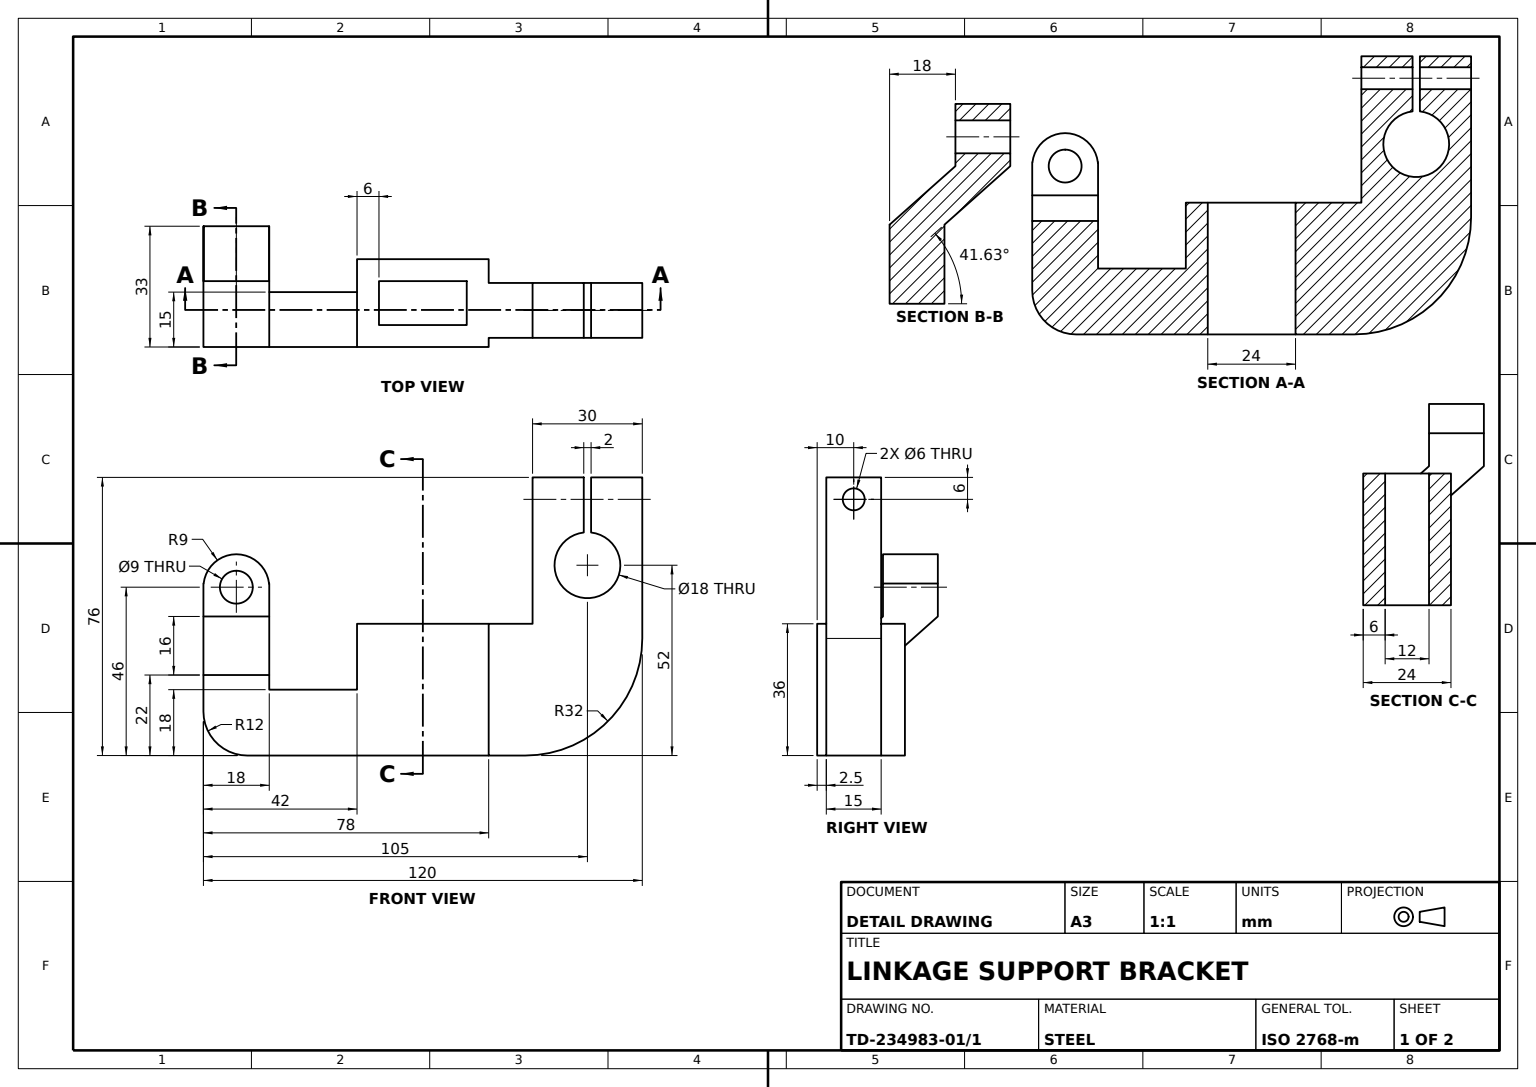
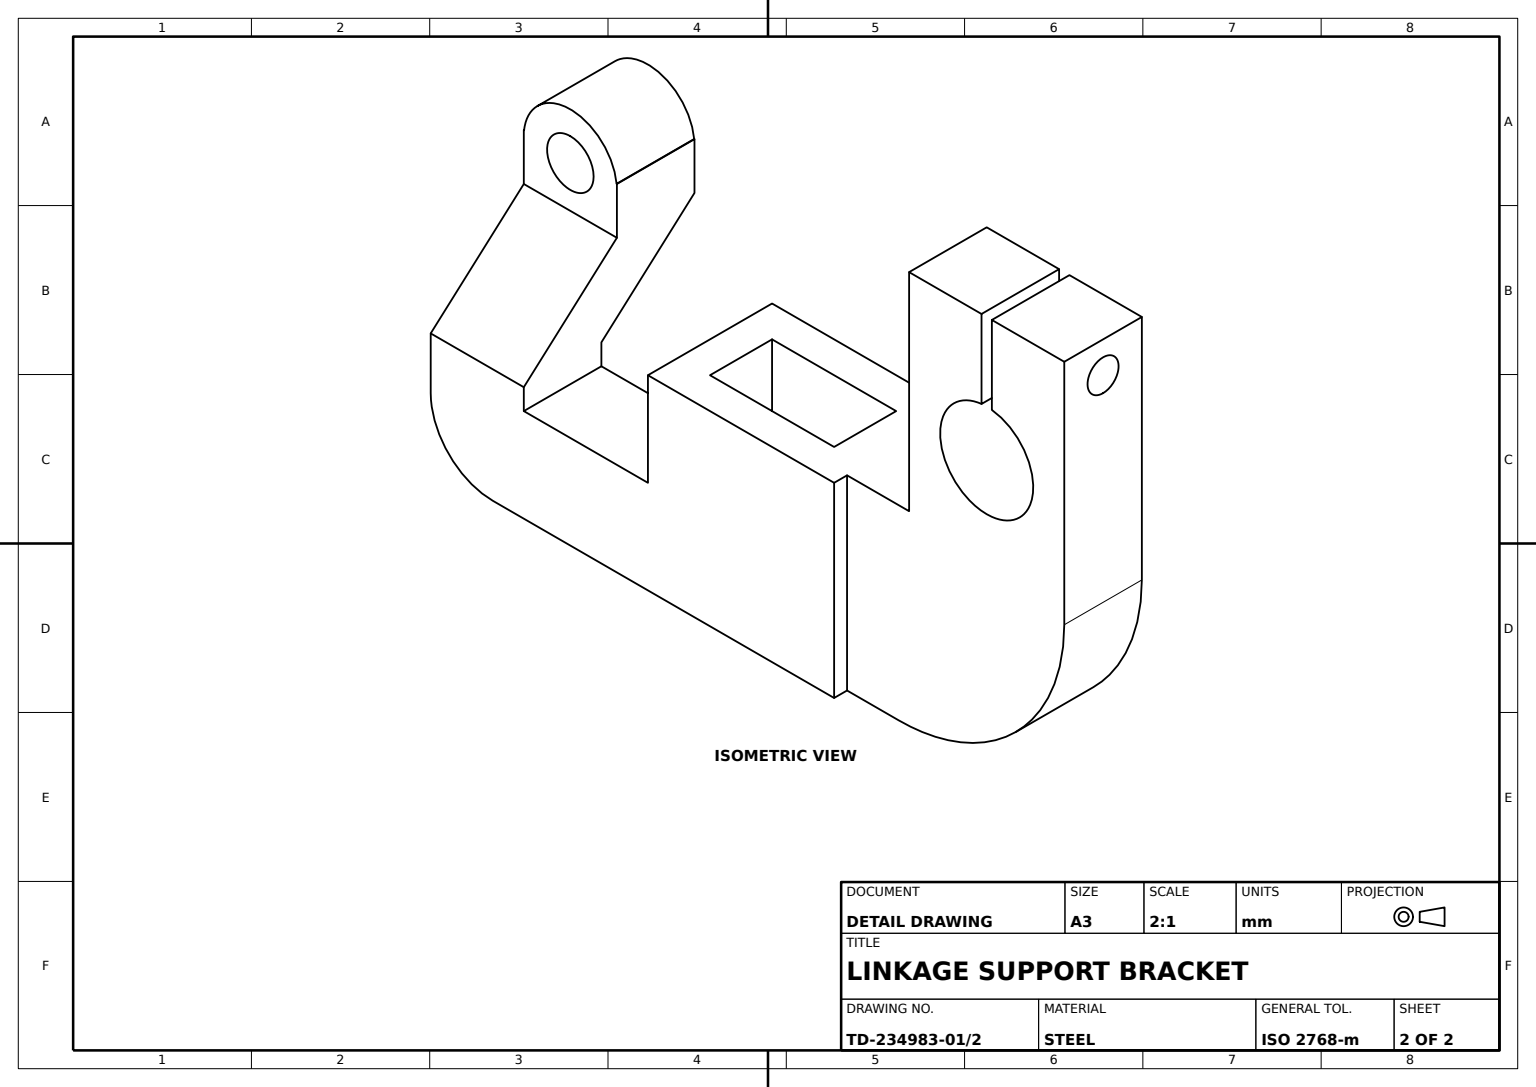
ISO-10303-21;
HEADER;
FILE_DESCRIPTION((''),'2;1');
FILE_NAME('','',(''),(''),'','','');
FILE_SCHEMA(('AUTOMOTIVE_DESIGN'));
ENDSEC;
DATA;
#1=APPLICATION_CONTEXT('');
#2=PRODUCT_CONTEXT('',#1,'mechanical');
#3=PRODUCT('','','',(#2));
#4=PRODUCT_DEFINITION_FORMATION('','',#3);
#5=PRODUCT_DEFINITION_CONTEXT('',#1,'design');
#6=PRODUCT_DEFINITION('','',#4,#5);
#7=PRODUCT_DEFINITION_SHAPE('','',#6);
#8=(LENGTH_UNIT()NAMED_UNIT(*)SI_UNIT(.MILLI.,.METRE.));
#9=(NAMED_UNIT(*)PLANE_ANGLE_UNIT()SI_UNIT($,.RADIAN.));
#10=(NAMED_UNIT(*)SI_UNIT($,.STERADIAN.)SOLID_ANGLE_UNIT());
#11=UNCERTAINTY_MEASURE_WITH_UNIT(LENGTH_MEASURE(0.005),#8,'distance_accuracy_value','');
#12=(GEOMETRIC_REPRESENTATION_CONTEXT(3)GLOBAL_UNCERTAINTY_ASSIGNED_CONTEXT((#11))GLOBAL_UNIT_ASSIGNED_CONTEXT((#8,#9,#10))REPRESENTATION_CONTEXT('',''));
#13=CARTESIAN_POINT('',(-16.5,18.,0.));
#14=VERTEX_POINT('',#13);
#15=CARTESIAN_POINT('',(-16.5,-18.,0.));
#16=VERTEX_POINT('',#15);
#17=DIRECTION('',(0.,-1.,0.));
#18=VECTOR('',#17,1000.);
#19=LINE('',#13,#18);
#20=EDGE_CURVE('',#14,#16,#19,.T.);
#21=ORIENTED_EDGE('',*,*,#20,.T.);
#22=CARTESIAN_POINT('',(-16.5,-18.,36.));
#23=VERTEX_POINT('',#22);
#24=DIRECTION('',(0.,0.,1.));
#25=VECTOR('',#24,1000.);
#26=LINE('',#15,#25);
#27=EDGE_CURVE('',#16,#23,#26,.T.);
#28=ORIENTED_EDGE('',*,*,#27,.T.);
#29=CARTESIAN_POINT('',(-16.5,18.,36.));
#30=VERTEX_POINT('',#29);
#31=DIRECTION('',(0.,1.,0.));
#32=VECTOR('',#31,1000.);
#33=LINE('',#22,#32);
#34=EDGE_CURVE('',#23,#30,#33,.T.);
#35=ORIENTED_EDGE('',*,*,#34,.T.);
#36=DIRECTION('',(0.,0.,-1.));
#37=VECTOR('',#36,1000.);
#38=LINE('',#29,#37);
#39=EDGE_CURVE('',#30,#14,#38,.T.);
#40=ORIENTED_EDGE('',*,*,#39,.T.);
#41=EDGE_LOOP('',(#21,#28,#35,#40));
#42=FACE_BOUND('',#41,.T.);
#43=CARTESIAN_POINT('',(-16.5,0.,0.));
#44=DIRECTION('',(-1.,0.,0.));
#45=AXIS2_PLACEMENT_3D('',#43,#44,#24);
#46=PLANE('',#45);
#47=ADVANCED_FACE('',(#42),#46,.T.);
#48=CARTESIAN_POINT('',(-25.5,-42.055728,47.));
#49=VERTEX_POINT('',#48);
#50=CARTESIAN_POINT('',(-25.5,-42.,47.));
#51=VERTEX_POINT('',#50);
#52=CARTESIAN_POINT('',(-25.5,-60.,47.));
#53=LINE('',#52,#32);
#54=EDGE_CURVE('',#49,#51,#53,.T.);
#55=ORIENTED_EDGE('',*,*,#54,.T.);
#56=CARTESIAN_POINT('',(-25.5,-42.,38.));
#57=VERTEX_POINT('',#56);
#58=LINE('',#56,#25);
#59=EDGE_CURVE('',#57,#51,#58,.T.);
#60=ORIENTED_EDGE('',*,*,#59,.F.);
#61=CARTESIAN_POINT('',(-25.5,-60.,38.));
#62=VERTEX_POINT('',#61);
#63=LINE('',#61,#32);
#64=EDGE_CURVE('',#62,#57,#63,.T.);
#65=ORIENTED_EDGE('',*,*,#64,.F.);
#66=VERTEX_POINT('',#52);
#67=LINE('',#61,#25);
#68=EDGE_CURVE('',#62,#66,#67,.T.);
#69=ORIENTED_EDGE('',*,*,#68,.T.);
#70=CARTESIAN_POINT('',(-25.5,-59.944272,47.));
#71=VERTEX_POINT('',#70);
#72=EDGE_CURVE('',#66,#71,#53,.T.);
#73=ORIENTED_EDGE('',*,*,#72,.T.);
#74=CARTESIAN_POINT('',(-25.5,-51.,46.));
#75=DIRECTION('',(1.,0.,0.));
#76=AXIS2_PLACEMENT_3D('',#74,#75,#31);
#77=CIRCLE('',#76,9.);
#78=EDGE_CURVE('',#49,#71,#77,.T.);
#79=ORIENTED_EDGE('',*,*,#78,.F.);
#80=EDGE_LOOP('',(#55,#60,#65,#69,#73,#79));
#81=FACE_BOUND('',#80,.T.);
#82=CARTESIAN_POINT('',(-25.5,-51.,50.5));
#83=VERTEX_POINT('',#82);
#84=AXIS2_PLACEMENT_3D('',#74,#44,#24);
#85=CIRCLE('',#84,4.5);
#86=EDGE_CURVE('',#83,#83,#85,.T.);
#87=ORIENTED_EDGE('',*,*,#86,.F.);
#88=EDGE_LOOP('',(#87));
#89=FACE_BOUND('',#88,.T.);
#90=AXIS2_PLACEMENT_3D('',#61,#44,#24);
#91=PLANE('',#90);
#92=ADVANCED_FACE('',(#81,#89),#91,.T.);
#93=CARTESIAN_POINT('',(-10.,44.,76.));
#94=VERTEX_POINT('',#93);
#95=CARTESIAN_POINT('',(-10.,30.,76.));
#96=VERTEX_POINT('',#95);
#97=CARTESIAN_POINT('',(-10.,60.,76.));
#98=LINE('',#97,#18);
#99=EDGE_CURVE('',#94,#96,#98,.T.);
#100=ORIENTED_EDGE('',*,*,#99,.T.);
#101=CARTESIAN_POINT('',(5.,30.,76.));
#102=VERTEX_POINT('',#101);
#103=VECTOR('',#44,1000.);
#104=LINE('',#101,#103);
#105=EDGE_CURVE('',#102,#96,#104,.T.);
#106=ORIENTED_EDGE('',*,*,#105,.F.);
#107=CARTESIAN_POINT('',(5.,44.,76.));
#108=VERTEX_POINT('',#107);
#109=CARTESIAN_POINT('',(5.,60.,76.));
#110=LINE('',#109,#18);
#111=EDGE_CURVE('',#108,#102,#110,.T.);
#112=ORIENTED_EDGE('',*,*,#111,.F.);
#113=VECTOR('',#75,1000.);
#114=LINE('',#107,#113);
#115=EDGE_CURVE('',#94,#108,#114,.T.);
#116=ORIENTED_EDGE('',*,*,#115,.F.);
#117=EDGE_LOOP('',(#100,#106,#112,#116));
#118=FACE_BOUND('',#117,.T.);
#119=AXIS2_PLACEMENT_3D('',#109,#36,#44);
#120=PLANE('',#119);
#121=ADVANCED_FACE('',(#118),#120,.F.);
#122=CARTESIAN_POINT('',(7.5,18.,36.));
#123=VERTEX_POINT('',#122);
#124=CARTESIAN_POINT('',(7.5,18.,0.));
#125=VERTEX_POINT('',#124);
#126=CARTESIAN_POINT('',(7.5,18.,18.));
#127=LINE('',#126,#37);
#128=EDGE_CURVE('',#123,#125,#127,.T.);
#129=ORIENTED_EDGE('',*,*,#128,.T.);
#130=CARTESIAN_POINT('',(5.,18.,0.));
#131=VERTEX_POINT('',#130);
#132=CARTESIAN_POINT('',(-7.5,18.,0.));
#133=LINE('',#132,#113);
#134=EDGE_CURVE('',#131,#125,#133,.T.);
#135=ORIENTED_EDGE('',*,*,#134,.F.);
#136=CARTESIAN_POINT('',(5.,18.,36.));
#137=VERTEX_POINT('',#136);
#138=LINE('',#130,#25);
#139=EDGE_CURVE('',#131,#137,#138,.T.);
#140=ORIENTED_EDGE('',*,*,#139,.T.);
#141=LINE('',#122,#103);
#142=EDGE_CURVE('',#123,#137,#141,.T.);
#143=ORIENTED_EDGE('',*,*,#142,.F.);
#144=EDGE_LOOP('',(#129,#135,#140,#143));
#145=FACE_BOUND('',#144,.T.);
#146=CARTESIAN_POINT('',(-7.5,18.,18.));
#147=AXIS2_PLACEMENT_3D('',#146,#17,#36);
#148=PLANE('',#147);
#149=ADVANCED_FACE('',(#145),#148,.F.);
#150=CARTESIAN_POINT('',(-10.5,-59.944272,47.));
#151=VERTEX_POINT('',#150);
#152=LINE('',#70,#113);
#153=EDGE_CURVE('',#71,#151,#152,.T.);
#154=ORIENTED_EDGE('',*,*,#153,.T.);
#155=CARTESIAN_POINT('',(-10.5,-42.055728,47.));
#156=VERTEX_POINT('',#155);
#157=CARTESIAN_POINT('',(-10.5,-51.,46.));
#158=AXIS2_PLACEMENT_3D('',#157,#75,#31);
#159=CIRCLE('',#158,9.);
#160=EDGE_CURVE('',#156,#151,#159,.T.);
#161=ORIENTED_EDGE('',*,*,#160,.F.);
#162=LINE('',#48,#113);
#163=EDGE_CURVE('',#156,#49,#162,.F.);
#164=ORIENTED_EDGE('',*,*,#163,.T.);
#165=ORIENTED_EDGE('',*,*,#78,.T.);
#166=EDGE_LOOP('',(#154,#161,#164,#165));
#167=FACE_BOUND('',#166,.T.);
#168=AXIS2_PLACEMENT_3D('',#74,#75,#36);
#169=CYLINDRICAL_SURFACE('',#168,9.);
#170=ADVANCED_FACE('',(#167),#169,.T.);
#171=VERTEX_POINT('',#97);
#172=CARTESIAN_POINT('',(-10.,46.,76.));
#173=VERTEX_POINT('',#172);
#174=EDGE_CURVE('',#171,#173,#98,.T.);
#175=ORIENTED_EDGE('',*,*,#174,.T.);
#176=CARTESIAN_POINT('',(5.,46.,76.));
#177=VERTEX_POINT('',#176);
#178=LINE('',#176,#103);
#179=EDGE_CURVE('',#177,#173,#178,.T.);
#180=ORIENTED_EDGE('',*,*,#179,.F.);
#181=VERTEX_POINT('',#109);
#182=EDGE_CURVE('',#181,#177,#110,.T.);
#183=ORIENTED_EDGE('',*,*,#182,.F.);
#184=LINE('',#109,#103);
#185=EDGE_CURVE('',#181,#171,#184,.T.);
#186=ORIENTED_EDGE('',*,*,#185,.T.);
#187=EDGE_LOOP('',(#175,#180,#183,#186));
#188=FACE_BOUND('',#187,.T.);
#189=ADVANCED_FACE('',(#188),#120,.F.);
#190=CARTESIAN_POINT('',(-2.5,44.,73.));
#191=VERTEX_POINT('',#190);
#192=CARTESIAN_POINT('',(-2.5,44.,70.));
#193=AXIS2_PLACEMENT_3D('',#192,#31,#24);
#194=CIRCLE('',#193,3.);
#195=EDGE_CURVE('',#191,#191,#194,.T.);
#196=ORIENTED_EDGE('',*,*,#195,.T.);
#197=EDGE_LOOP('',(#196));
#198=FACE_BOUND('',#197,.T.);
#199=CARTESIAN_POINT('',(-2.5,30.,73.));
#200=VERTEX_POINT('',#199);
#201=CARTESIAN_POINT('',(-2.5,30.,70.));
#202=AXIS2_PLACEMENT_3D('',#201,#31,#24);
#203=CIRCLE('',#202,3.);
#204=EDGE_CURVE('',#200,#200,#203,.T.);
#205=ORIENTED_EDGE('',*,*,#204,.F.);
#206=EDGE_LOOP('',(#205));
#207=FACE_BOUND('',#206,.T.);
#208=CYLINDRICAL_SURFACE('',#202,3.);
#209=ADVANCED_FACE('',(#198,#207),#208,.F.);
#210=ORIENTED_EDGE('',*,*,#59,.T.);
#211=CARTESIAN_POINT('',(-10.5,-42.,47.));
#212=VERTEX_POINT('',#211);
#213=LINE('',#50,#113);
#214=EDGE_CURVE('',#51,#212,#213,.T.);
#215=ORIENTED_EDGE('',*,*,#214,.T.);
#216=CARTESIAN_POINT('',(-10.5,-42.,38.));
#217=VERTEX_POINT('',#216);
#218=LINE('',#211,#37);
#219=EDGE_CURVE('',#212,#217,#218,.T.);
#220=ORIENTED_EDGE('',*,*,#219,.T.);
#221=CARTESIAN_POINT('',(7.5,-42.,22.));
#222=VERTEX_POINT('',#221);
#223=DIRECTION('',(0.747409319,0.,-0.664363839));
#224=VECTOR('',#223,1000.);
#225=LINE('',#216,#224);
#226=EDGE_CURVE('',#217,#222,#225,.T.);
#227=ORIENTED_EDGE('',*,*,#226,.T.);
#228=CARTESIAN_POINT('',(7.5,-42.,18.));
#229=VERTEX_POINT('',#228);
#230=CARTESIAN_POINT('',(7.5,-42.,0.));
#231=LINE('',#230,#25);
#232=EDGE_CURVE('',#229,#222,#231,.T.);
#233=ORIENTED_EDGE('',*,*,#232,.F.);
#234=CARTESIAN_POINT('',(-7.5,-42.,18.));
#235=VERTEX_POINT('',#234);
#236=LINE('',#234,#103);
#237=EDGE_CURVE('',#229,#235,#236,.T.);
#238=ORIENTED_EDGE('',*,*,#237,.T.);
#239=CARTESIAN_POINT('',(-7.5,-42.,22.));
#240=VERTEX_POINT('',#239);
#241=CARTESIAN_POINT('',(-7.5,-42.,0.));
#242=LINE('',#241,#25);
#243=EDGE_CURVE('',#235,#240,#242,.T.);
#244=ORIENTED_EDGE('',*,*,#243,.T.);
#245=DIRECTION('',(-0.747409319,0.,0.664363839));
#246=VECTOR('',#245,1000.);
#247=LINE('',#239,#246);
#248=EDGE_CURVE('',#240,#57,#247,.T.);
#249=ORIENTED_EDGE('',*,*,#248,.T.);
#250=EDGE_LOOP('',(#210,#215,#220,#227,#233,#238,#244,#249));
#251=FACE_BOUND('',#250,.T.);
#252=AXIS2_PLACEMENT_3D('',#230,#17,#36);
#253=PLANE('',#252);
#254=ADVANCED_FACE('',(#251),#253,.F.);
#255=CARTESIAN_POINT('',(-10.5,-12.,36.));
#256=VERTEX_POINT('',#255);
#257=CARTESIAN_POINT('',(-10.5,12.,36.));
#258=VERTEX_POINT('',#257);
#259=CARTESIAN_POINT('',(-10.5,18.,36.));
#260=LINE('',#259,#32);
#261=EDGE_CURVE('',#256,#258,#260,.T.);
#262=ORIENTED_EDGE('',*,*,#261,.F.);
#263=CARTESIAN_POINT('',(-10.5,-12.,0.));
#264=VERTEX_POINT('',#263);
#265=CARTESIAN_POINT('',(-10.5,-12.,51.));
#266=LINE('',#265,#37);
#267=EDGE_CURVE('',#264,#256,#266,.F.);
#268=ORIENTED_EDGE('',*,*,#267,.F.);
#269=CARTESIAN_POINT('',(-10.5,12.,0.));
#270=VERTEX_POINT('',#269);
#271=CARTESIAN_POINT('',(-10.5,18.,0.));
#272=LINE('',#271,#32);
#273=EDGE_CURVE('',#264,#270,#272,.T.);
#274=ORIENTED_EDGE('',*,*,#273,.T.);
#275=CARTESIAN_POINT('',(-10.5,12.,51.));
#276=LINE('',#275,#37);
#277=EDGE_CURVE('',#270,#258,#276,.F.);
#278=ORIENTED_EDGE('',*,*,#277,.T.);
#279=EDGE_LOOP('',(#262,#268,#274,#278));
#280=FACE_BOUND('',#279,.T.);
#281=AXIS2_PLACEMENT_3D('',#275,#75,#31);
#282=PLANE('',#281);
#283=ADVANCED_FACE('',(#280),#282,.T.);
#284=CARTESIAN_POINT('',(-10.5,-60.,38.));
#285=VERTEX_POINT('',#284);
#286=CARTESIAN_POINT('',(7.5,-60.,22.));
#287=VERTEX_POINT('',#286);
#288=LINE('',#284,#224);
#289=EDGE_CURVE('',#285,#287,#288,.T.);
#290=ORIENTED_EDGE('',*,*,#289,.F.);
#291=CARTESIAN_POINT('',(-10.5,-60.,47.));
#292=VERTEX_POINT('',#291);
#293=LINE('',#291,#37);
#294=EDGE_CURVE('',#292,#285,#293,.T.);
#295=ORIENTED_EDGE('',*,*,#294,.F.);
#296=LINE('',#52,#113);
#297=EDGE_CURVE('',#66,#292,#296,.T.);
#298=ORIENTED_EDGE('',*,*,#297,.F.);
#299=ORIENTED_EDGE('',*,*,#68,.F.);
#300=CARTESIAN_POINT('',(-7.5,-60.,22.));
#301=VERTEX_POINT('',#300);
#302=LINE('',#300,#246);
#303=EDGE_CURVE('',#301,#62,#302,.T.);
#304=ORIENTED_EDGE('',*,*,#303,.F.);
#305=CARTESIAN_POINT('',(-7.5,-60.,12.));
#306=VERTEX_POINT('',#305);
#307=CARTESIAN_POINT('',(-7.5,-60.,0.));
#308=LINE('',#307,#25);
#309=EDGE_CURVE('',#306,#301,#308,.T.);
#310=ORIENTED_EDGE('',*,*,#309,.F.);
#311=CARTESIAN_POINT('',(7.5,-60.,12.));
#312=VERTEX_POINT('',#311);
#313=LINE('',#305,#113);
#314=EDGE_CURVE('',#306,#312,#313,.T.);
#315=ORIENTED_EDGE('',*,*,#314,.T.);
#316=CARTESIAN_POINT('',(7.5,-60.,0.));
#317=LINE('',#316,#25);
#318=EDGE_CURVE('',#312,#287,#317,.T.);
#319=ORIENTED_EDGE('',*,*,#318,.T.);
#320=EDGE_LOOP('',(#290,#295,#298,#299,#304,#310,#315,#319));
#321=FACE_BOUND('',#320,.T.);
#322=AXIS2_PLACEMENT_3D('',#307,#31,#24);
#323=PLANE('',#322);
#324=ADVANCED_FACE('',(#321),#323,.F.);
#325=ORIENTED_EDGE('',*,*,#72,.F.);
#326=ORIENTED_EDGE('',*,*,#297,.T.);
#327=LINE('',#291,#32);
#328=EDGE_CURVE('',#292,#151,#327,.T.);
#329=ORIENTED_EDGE('',*,*,#328,.T.);
#330=ORIENTED_EDGE('',*,*,#153,.F.);
#331=EDGE_LOOP('',(#325,#326,#329,#330));
#332=FACE_BOUND('',#331,.T.);
#333=AXIS2_PLACEMENT_3D('',#52,#24,#75);
#334=PLANE('',#333);
#335=ADVANCED_FACE('',(#332),#334,.T.);
#336=ORIENTED_EDGE('',*,*,#277,.F.);
#337=CARTESIAN_POINT('',(1.5,12.,0.));
#338=VERTEX_POINT('',#337);
#339=CARTESIAN_POINT('',(-7.5,12.,0.));
#340=LINE('',#339,#113);
#341=EDGE_CURVE('',#270,#338,#340,.T.);
#342=ORIENTED_EDGE('',*,*,#341,.T.);
#343=CARTESIAN_POINT('',(1.5,12.,36.));
#344=VERTEX_POINT('',#343);
#345=CARTESIAN_POINT('',(1.5,12.,51.));
#346=LINE('',#345,#37);
#347=EDGE_CURVE('',#338,#344,#346,.F.);
#348=ORIENTED_EDGE('',*,*,#347,.T.);
#349=CARTESIAN_POINT('',(5.,12.,36.));
#350=LINE('',#349,#113);
#351=EDGE_CURVE('',#258,#344,#350,.T.);
#352=ORIENTED_EDGE('',*,*,#351,.F.);
#353=EDGE_LOOP('',(#336,#342,#348,#352));
#354=FACE_BOUND('',#353,.T.);
#355=AXIS2_PLACEMENT_3D('',#345,#17,#36);
#356=PLANE('',#355);
#357=ADVANCED_FACE('',(#354),#356,.T.);
#358=ORIENTED_EDGE('',*,*,#204,.T.);
#359=EDGE_LOOP('',(#358));
#360=FACE_BOUND('',#359,.T.);
#361=CARTESIAN_POINT('',(-10.,30.,36.));
#362=VERTEX_POINT('',#361);
#363=LINE('',#95,#37);
#364=EDGE_CURVE('',#362,#96,#363,.F.);
#365=ORIENTED_EDGE('',*,*,#364,.F.);
#366=CARTESIAN_POINT('',(5.,30.,36.));
#367=VERTEX_POINT('',#366);
#368=LINE('',#366,#103);
#369=EDGE_CURVE('',#367,#362,#368,.T.);
#370=ORIENTED_EDGE('',*,*,#369,.F.);
#371=LINE('',#101,#37);
#372=EDGE_CURVE('',#102,#367,#371,.T.);
#373=ORIENTED_EDGE('',*,*,#372,.F.);
#374=ORIENTED_EDGE('',*,*,#105,.T.);
#375=EDGE_LOOP('',(#365,#370,#373,#374));
#376=FACE_BOUND('',#375,.T.);
#377=AXIS2_PLACEMENT_3D('',#101,#31,#24);
#378=PLANE('',#377);
#379=ADVANCED_FACE('',(#360,#376),#378,.F.);
#380=CARTESIAN_POINT('',(-10.,18.,36.));
#381=VERTEX_POINT('',#380);
#382=LINE('',#380,#32);
#383=EDGE_CURVE('',#381,#362,#382,.T.);
#384=ORIENTED_EDGE('',*,*,#383,.T.);
#385=ORIENTED_EDGE('',*,*,#364,.T.);
#386=ORIENTED_EDGE('',*,*,#99,.F.);
#387=CARTESIAN_POINT('',(-10.,44.,60.944272));
#388=VERTEX_POINT('',#387);
#389=CARTESIAN_POINT('',(-10.,44.,0.));
#390=LINE('',#389,#37);
#391=EDGE_CURVE('',#94,#388,#390,.T.);
#392=ORIENTED_EDGE('',*,*,#391,.T.);
#393=CARTESIAN_POINT('',(-10.,46.,60.944272));
#394=VERTEX_POINT('',#393);
#395=CARTESIAN_POINT('',(-10.,45.,52.));
#396=AXIS2_PLACEMENT_3D('',#395,#44,#24);
#397=CIRCLE('',#396,9.);
#398=EDGE_CURVE('',#394,#388,#397,.T.);
#399=ORIENTED_EDGE('',*,*,#398,.F.);
#400=CARTESIAN_POINT('',(-10.,46.,0.));
#401=LINE('',#400,#25);
#402=EDGE_CURVE('',#394,#173,#401,.T.);
#403=ORIENTED_EDGE('',*,*,#402,.T.);
#404=ORIENTED_EDGE('',*,*,#174,.F.);
#405=CARTESIAN_POINT('',(-10.,60.,32.));
#406=VERTEX_POINT('',#405);
#407=CARTESIAN_POINT('',(-10.,60.,0.));
#408=LINE('',#407,#25);
#409=EDGE_CURVE('',#406,#171,#408,.T.);
#410=ORIENTED_EDGE('',*,*,#409,.F.);
#411=CARTESIAN_POINT('',(-10.,28.,0.));
#412=VERTEX_POINT('',#411);
#413=CARTESIAN_POINT('',(-10.,28.,32.));
#414=AXIS2_PLACEMENT_3D('',#413,#44,#24);
#415=CIRCLE('',#414,32.);
#416=EDGE_CURVE('',#406,#412,#415,.T.);
#417=ORIENTED_EDGE('',*,*,#416,.T.);
#418=CARTESIAN_POINT('',(-10.,18.,0.));
#419=VERTEX_POINT('',#418);
#420=CARTESIAN_POINT('',(-10.,33.454545,0.));
#421=LINE('',#420,#18);
#422=EDGE_CURVE('',#412,#419,#421,.T.);
#423=ORIENTED_EDGE('',*,*,#422,.T.);
#424=LINE('',#418,#25);
#425=EDGE_CURVE('',#419,#381,#424,.T.);
#426=ORIENTED_EDGE('',*,*,#425,.T.);
#427=EDGE_LOOP('',(#384,#385,#386,#392,#399,#403,#404,#410,#417,#423,#426));
#428=FACE_BOUND('',#427,.T.);
#429=CARTESIAN_POINT('',(-10.,0.,0.));
#430=AXIS2_PLACEMENT_3D('',#429,#44,#24);
#431=PLANE('',#430);
#432=ADVANCED_FACE('',(#428),#431,.T.);
#433=CARTESIAN_POINT('',(7.5,-48.,0.));
#434=VERTEX_POINT('',#433);
#435=CARTESIAN_POINT('',(7.5,-48.,12.));
#436=AXIS2_PLACEMENT_3D('',#435,#44,#24);
#437=CIRCLE('',#436,12.);
#438=EDGE_CURVE('',#312,#434,#437,.F.);
#439=ORIENTED_EDGE('',*,*,#438,.F.);
#440=ORIENTED_EDGE('',*,*,#314,.F.);
#441=CARTESIAN_POINT('',(-7.5,-48.,0.));
#442=VERTEX_POINT('',#441);
#443=CARTESIAN_POINT('',(-7.5,-48.,12.));
#444=AXIS2_PLACEMENT_3D('',#443,#44,#24);
#445=CIRCLE('',#444,12.);
#446=EDGE_CURVE('',#442,#306,#445,.T.);
#447=ORIENTED_EDGE('',*,*,#446,.F.);
#448=LINE('',#441,#113);
#449=EDGE_CURVE('',#434,#442,#448,.F.);
#450=ORIENTED_EDGE('',*,*,#449,.F.);
#451=EDGE_LOOP('',(#439,#440,#447,#450));
#452=FACE_BOUND('',#451,.T.);
#453=AXIS2_PLACEMENT_3D('',#443,#75,#36);
#454=CYLINDRICAL_SURFACE('',#453,12.);
#455=ADVANCED_FACE('',(#452),#454,.T.);
#456=CARTESIAN_POINT('',(-2.5,46.,67.));
#457=VERTEX_POINT('',#456);
#458=CARTESIAN_POINT('',(-2.5,46.,70.));
#459=AXIS2_PLACEMENT_3D('',#458,#17,#36);
#460=CIRCLE('',#459,3.);
#461=EDGE_CURVE('',#457,#457,#460,.T.);
#462=ORIENTED_EDGE('',*,*,#461,.F.);
#463=EDGE_LOOP('',(#462));
#464=FACE_BOUND('',#463,.T.);
#465=CARTESIAN_POINT('',(5.,46.,60.944272));
#466=VERTEX_POINT('',#465);
#467=LINE('',#465,#103);
#468=EDGE_CURVE('',#466,#394,#467,.T.);
#469=ORIENTED_EDGE('',*,*,#468,.F.);
#470=CARTESIAN_POINT('',(5.,46.,0.));
#471=LINE('',#470,#25);
#472=EDGE_CURVE('',#466,#177,#471,.T.);
#473=ORIENTED_EDGE('',*,*,#472,.T.);
#474=ORIENTED_EDGE('',*,*,#179,.T.);
#475=ORIENTED_EDGE('',*,*,#402,.F.);
#476=EDGE_LOOP('',(#469,#473,#474,#475));
#477=FACE_BOUND('',#476,.T.);
#478=CARTESIAN_POINT('',(14.5,46.,85.));
#479=AXIS2_PLACEMENT_3D('',#478,#17,#36);
#480=PLANE('',#479);
#481=ADVANCED_FACE('',(#464,#477),#480,.T.);
#482=CARTESIAN_POINT('',(-7.5,-18.,0.));
#483=VERTEX_POINT('',#482);
#484=CARTESIAN_POINT('',(-7.5,-18.,18.));
#485=VERTEX_POINT('',#484);
#486=LINE('',#482,#25);
#487=EDGE_CURVE('',#483,#485,#486,.T.);
#488=ORIENTED_EDGE('',*,*,#487,.F.);
#489=LINE('',#132,#18);
#490=EDGE_CURVE('',#483,#442,#489,.T.);
#491=ORIENTED_EDGE('',*,*,#490,.T.);
#492=ORIENTED_EDGE('',*,*,#446,.T.);
#493=ORIENTED_EDGE('',*,*,#309,.T.);
#494=LINE('',#239,#18);
#495=EDGE_CURVE('',#240,#301,#494,.T.);
#496=ORIENTED_EDGE('',*,*,#495,.F.);
#497=ORIENTED_EDGE('',*,*,#243,.F.);
#498=CARTESIAN_POINT('',(-7.5,-60.,18.));
#499=LINE('',#498,#32);
#500=EDGE_CURVE('',#235,#485,#499,.T.);
#501=ORIENTED_EDGE('',*,*,#500,.T.);
#502=EDGE_LOOP('',(#488,#491,#492,#493,#496,#497,#501));
#503=FACE_BOUND('',#502,.T.);
#504=CARTESIAN_POINT('',(-7.5,0.,0.));
#505=AXIS2_PLACEMENT_3D('',#504,#44,#24);
#506=PLANE('',#505);
#507=ADVANCED_FACE('',(#503),#506,.T.);
#508=CARTESIAN_POINT('',(7.5,-18.,18.));
#509=VERTEX_POINT('',#508);
#510=LINE('',#484,#103);
#511=EDGE_CURVE('',#509,#485,#510,.T.);
#512=ORIENTED_EDGE('',*,*,#511,.F.);
#513=CARTESIAN_POINT('',(7.5,-18.,36.));
#514=VERTEX_POINT('',#513);
#515=CARTESIAN_POINT('',(7.5,-18.,0.));
#516=LINE('',#515,#25);
#517=EDGE_CURVE('',#514,#509,#516,.F.);
#518=ORIENTED_EDGE('',*,*,#517,.F.);
#519=LINE('',#513,#103);
#520=EDGE_CURVE('',#514,#23,#519,.T.);
#521=ORIENTED_EDGE('',*,*,#520,.T.);
#522=ORIENTED_EDGE('',*,*,#27,.F.);
#523=LINE('',#515,#103);
#524=EDGE_CURVE('',#483,#16,#523,.T.);
#525=ORIENTED_EDGE('',*,*,#524,.F.);
#526=ORIENTED_EDGE('',*,*,#487,.T.);
#527=EDGE_LOOP('',(#512,#518,#521,#522,#525,#526));
#528=FACE_BOUND('',#527,.T.);
#529=AXIS2_PLACEMENT_3D('',#515,#17,#36);
#530=PLANE('',#529);
#531=ADVANCED_FACE('',(#528),#530,.T.);
#532=EDGE_CURVE('',#381,#30,#141,.T.);
#533=ORIENTED_EDGE('',*,*,#532,.F.);
#534=ORIENTED_EDGE('',*,*,#425,.F.);
#535=LINE('',#124,#103);
#536=EDGE_CURVE('',#419,#14,#535,.T.);
#537=ORIENTED_EDGE('',*,*,#536,.T.);
#538=ORIENTED_EDGE('',*,*,#39,.F.);
#539=EDGE_LOOP('',(#533,#534,#537,#538));
#540=FACE_BOUND('',#539,.T.);
#541=AXIS2_PLACEMENT_3D('',#122,#31,#24);
#542=PLANE('',#541);
#543=ADVANCED_FACE('',(#540),#542,.T.);
#544=ORIENTED_EDGE('',*,*,#139,.F.);
#545=CARTESIAN_POINT('',(5.,28.,0.));
#546=VERTEX_POINT('',#545);
#547=CARTESIAN_POINT('',(5.,33.454545,0.));
#548=LINE('',#547,#18);
#549=EDGE_CURVE('',#546,#131,#548,.T.);
#550=ORIENTED_EDGE('',*,*,#549,.F.);
#551=CARTESIAN_POINT('',(5.,60.,32.));
#552=VERTEX_POINT('',#551);
#553=CARTESIAN_POINT('',(5.,28.,32.));
#554=AXIS2_PLACEMENT_3D('',#553,#44,#24);
#555=CIRCLE('',#554,32.);
#556=EDGE_CURVE('',#546,#552,#555,.F.);
#557=ORIENTED_EDGE('',*,*,#556,.T.);
#558=CARTESIAN_POINT('',(5.,60.,0.));
#559=LINE('',#558,#25);
#560=EDGE_CURVE('',#552,#181,#559,.T.);
#561=ORIENTED_EDGE('',*,*,#560,.T.);
#562=ORIENTED_EDGE('',*,*,#182,.T.);
#563=ORIENTED_EDGE('',*,*,#472,.F.);
#564=CARTESIAN_POINT('',(5.,44.,60.944272));
#565=VERTEX_POINT('',#564);
#566=CARTESIAN_POINT('',(5.,45.,52.));
#567=AXIS2_PLACEMENT_3D('',#566,#44,#24);
#568=CIRCLE('',#567,9.);
#569=EDGE_CURVE('',#466,#565,#568,.T.);
#570=ORIENTED_EDGE('',*,*,#569,.T.);
#571=CARTESIAN_POINT('',(5.,44.,0.));
#572=LINE('',#571,#37);
#573=EDGE_CURVE('',#108,#565,#572,.T.);
#574=ORIENTED_EDGE('',*,*,#573,.F.);
#575=ORIENTED_EDGE('',*,*,#111,.T.);
#576=ORIENTED_EDGE('',*,*,#372,.T.);
#577=LINE('',#136,#32);
#578=EDGE_CURVE('',#137,#367,#577,.T.);
#579=ORIENTED_EDGE('',*,*,#578,.F.);
#580=EDGE_LOOP('',(#544,#550,#557,#561,#562,#563,#570,#574,#575,#576,#579));
#581=FACE_BOUND('',#580,.T.);
#582=CARTESIAN_POINT('',(5.,0.,0.));
#583=AXIS2_PLACEMENT_3D('',#582,#44,#24);
#584=PLANE('',#583);
#585=ADVANCED_FACE('',(#581),#584,.F.);
#586=CARTESIAN_POINT('',(-7.5,28.,0.));
#587=LINE('',#586,#103);
#588=EDGE_CURVE('',#412,#546,#587,.F.);
#589=ORIENTED_EDGE('',*,*,#588,.F.);
#590=ORIENTED_EDGE('',*,*,#416,.F.);
#591=LINE('',#551,#103);
#592=EDGE_CURVE('',#552,#406,#591,.T.);
#593=ORIENTED_EDGE('',*,*,#592,.F.);
#594=ORIENTED_EDGE('',*,*,#556,.F.);
#595=EDGE_LOOP('',(#589,#590,#593,#594));
#596=FACE_BOUND('',#595,.T.);
#597=CYLINDRICAL_SURFACE('',#554,32.);
#598=ADVANCED_FACE('',(#596),#597,.T.);
#599=ORIENTED_EDGE('',*,*,#328,.F.);
#600=ORIENTED_EDGE('',*,*,#294,.T.);
#601=LINE('',#284,#32);
#602=EDGE_CURVE('',#285,#217,#601,.T.);
#603=ORIENTED_EDGE('',*,*,#602,.T.);
#604=ORIENTED_EDGE('',*,*,#219,.F.);
#605=EDGE_CURVE('',#156,#212,#327,.T.);
#606=ORIENTED_EDGE('',*,*,#605,.F.);
#607=ORIENTED_EDGE('',*,*,#160,.T.);
#608=EDGE_LOOP('',(#599,#600,#603,#604,#606,#607));
#609=FACE_BOUND('',#608,.T.);
#610=CARTESIAN_POINT('',(-10.5,-51.,50.5));
#611=VERTEX_POINT('',#610);
#612=AXIS2_PLACEMENT_3D('',#157,#44,#24);
#613=CIRCLE('',#612,4.5);
#614=EDGE_CURVE('',#611,#611,#613,.T.);
#615=ORIENTED_EDGE('',*,*,#614,.T.);
#616=EDGE_LOOP('',(#615));
#617=FACE_BOUND('',#616,.T.);
#618=AXIS2_PLACEMENT_3D('',#291,#75,#36);
#619=PLANE('',#618);
#620=ADVANCED_FACE('',(#609,#617),#619,.T.);
#621=LINE('',#513,#32);
#622=EDGE_CURVE('',#514,#123,#621,.T.);
#623=ORIENTED_EDGE('',*,*,#622,.F.);
#624=ORIENTED_EDGE('',*,*,#517,.T.);
#625=CARTESIAN_POINT('',(7.5,-60.,18.));
#626=LINE('',#625,#32);
#627=EDGE_CURVE('',#229,#509,#626,.T.);
#628=ORIENTED_EDGE('',*,*,#627,.F.);
#629=ORIENTED_EDGE('',*,*,#232,.T.);
#630=LINE('',#221,#18);
#631=EDGE_CURVE('',#222,#287,#630,.T.);
#632=ORIENTED_EDGE('',*,*,#631,.T.);
#633=ORIENTED_EDGE('',*,*,#318,.F.);
#634=ORIENTED_EDGE('',*,*,#438,.T.);
#635=LINE('',#124,#18);
#636=EDGE_CURVE('',#125,#434,#635,.T.);
#637=ORIENTED_EDGE('',*,*,#636,.F.);
#638=ORIENTED_EDGE('',*,*,#128,.F.);
#639=EDGE_LOOP('',(#623,#624,#628,#629,#632,#633,#634,#637,#638));
#640=FACE_BOUND('',#639,.T.);
#641=CARTESIAN_POINT('',(7.5,0.,0.));
#642=AXIS2_PLACEMENT_3D('',#641,#44,#24);
#643=PLANE('',#642);
#644=ADVANCED_FACE('',(#640),#643,.F.);
#645=CARTESIAN_POINT('',(1.5,-12.,0.));
#646=VERTEX_POINT('',#645);
#647=CARTESIAN_POINT('',(-7.5,-12.,0.));
#648=LINE('',#647,#103);
#649=EDGE_CURVE('',#646,#264,#648,.T.);
#650=ORIENTED_EDGE('',*,*,#649,.T.);
#651=ORIENTED_EDGE('',*,*,#267,.T.);
#652=CARTESIAN_POINT('',(1.5,-12.,36.));
#653=VERTEX_POINT('',#652);
#654=CARTESIAN_POINT('',(5.,-12.,36.));
#655=LINE('',#654,#103);
#656=EDGE_CURVE('',#653,#256,#655,.T.);
#657=ORIENTED_EDGE('',*,*,#656,.F.);
#658=CARTESIAN_POINT('',(1.5,-12.,51.));
#659=LINE('',#658,#37);
#660=EDGE_CURVE('',#646,#653,#659,.F.);
#661=ORIENTED_EDGE('',*,*,#660,.F.);
#662=EDGE_LOOP('',(#650,#651,#657,#661));
#663=FACE_BOUND('',#662,.T.);
#664=AXIS2_PLACEMENT_3D('',#265,#31,#24);
#665=PLANE('',#664);
#666=ADVANCED_FACE('',(#663),#665,.T.);
#667=ORIENTED_EDGE('',*,*,#86,.T.);
#668=EDGE_LOOP('',(#667));
#669=FACE_BOUND('',#668,.T.);
#670=ORIENTED_EDGE('',*,*,#614,.F.);
#671=EDGE_LOOP('',(#670));
#672=FACE_BOUND('',#671,.T.);
#673=CYLINDRICAL_SURFACE('',#612,4.5);
#674=ADVANCED_FACE('',(#669,#672),#673,.F.);
#675=ORIENTED_EDGE('',*,*,#468,.T.);
#676=ORIENTED_EDGE('',*,*,#398,.T.);
#677=LINE('',#564,#103);
#678=EDGE_CURVE('',#388,#565,#677,.F.);
#679=ORIENTED_EDGE('',*,*,#678,.T.);
#680=ORIENTED_EDGE('',*,*,#569,.F.);
#681=EDGE_LOOP('',(#675,#676,#679,#680));
#682=FACE_BOUND('',#681,.T.);
#683=CYLINDRICAL_SURFACE('',#567,9.);
#684=ADVANCED_FACE('',(#682),#683,.F.);
#685=ORIENTED_EDGE('',*,*,#495,.T.);
#686=ORIENTED_EDGE('',*,*,#303,.T.);
#687=ORIENTED_EDGE('',*,*,#64,.T.);
#688=ORIENTED_EDGE('',*,*,#248,.F.);
#689=EDGE_LOOP('',(#685,#686,#687,#688));
#690=FACE_BOUND('',#689,.T.);
#691=DIRECTION('',(-0.664363839,0.,-0.747409319));
#692=AXIS2_PLACEMENT_3D('',#300,#691,#245);
#693=PLANE('',#692);
#694=ADVANCED_FACE('',(#690),#693,.T.);
#695=CARTESIAN_POINT('',(1.5,18.,0.));
#696=LINE('',#695,#18);
#697=EDGE_CURVE('',#338,#646,#696,.T.);
#698=ORIENTED_EDGE('',*,*,#697,.T.);
#699=ORIENTED_EDGE('',*,*,#660,.T.);
#700=CARTESIAN_POINT('',(1.5,18.,36.));
#701=LINE('',#700,#18);
#702=EDGE_CURVE('',#344,#653,#701,.T.);
#703=ORIENTED_EDGE('',*,*,#702,.F.);
#704=ORIENTED_EDGE('',*,*,#347,.F.);
#705=EDGE_LOOP('',(#698,#699,#703,#704));
#706=FACE_BOUND('',#705,.T.);
#707=AXIS2_PLACEMENT_3D('',#658,#44,#17);
#708=PLANE('',#707);
#709=ADVANCED_FACE('',(#706),#708,.T.);
#710=ORIENTED_EDGE('',*,*,#524,.T.);
#711=ORIENTED_EDGE('',*,*,#20,.F.);
#712=ORIENTED_EDGE('',*,*,#536,.F.);
#713=ORIENTED_EDGE('',*,*,#422,.F.);
#714=ORIENTED_EDGE('',*,*,#588,.T.);
#715=ORIENTED_EDGE('',*,*,#549,.T.);
#716=ORIENTED_EDGE('',*,*,#134,.T.);
#717=ORIENTED_EDGE('',*,*,#636,.T.);
#718=ORIENTED_EDGE('',*,*,#449,.T.);
#719=ORIENTED_EDGE('',*,*,#490,.F.);
#720=EDGE_LOOP('',(#710,#711,#712,#713,#714,#715,#716,#717,#718,#719));
#721=FACE_BOUND('',#720,.T.);
#722=ORIENTED_EDGE('',*,*,#273,.F.);
#723=ORIENTED_EDGE('',*,*,#649,.F.);
#724=ORIENTED_EDGE('',*,*,#697,.F.);
#725=ORIENTED_EDGE('',*,*,#341,.F.);
#726=EDGE_LOOP('',(#722,#723,#724,#725));
#727=FACE_BOUND('',#726,.T.);
#728=AXIS2_PLACEMENT_3D('',#132,#24,#75);
#729=PLANE('',#728);
#730=ADVANCED_FACE('',(#721,#727),#729,.F.);
#731=ORIENTED_EDGE('',*,*,#500,.F.);
#732=ORIENTED_EDGE('',*,*,#237,.F.);
#733=ORIENTED_EDGE('',*,*,#627,.T.);
#734=ORIENTED_EDGE('',*,*,#511,.T.);
#735=EDGE_LOOP('',(#731,#732,#733,#734));
#736=FACE_BOUND('',#735,.T.);
#737=AXIS2_PLACEMENT_3D('',#498,#36,#31);
#738=PLANE('',#737);
#739=ADVANCED_FACE('',(#736),#738,.F.);
#740=CARTESIAN_POINT('',(-2.5,60.,67.));
#741=VERTEX_POINT('',#740);
#742=CARTESIAN_POINT('',(-2.5,60.,70.));
#743=AXIS2_PLACEMENT_3D('',#742,#17,#36);
#744=CIRCLE('',#743,3.);
#745=EDGE_CURVE('',#741,#741,#744,.T.);
#746=ORIENTED_EDGE('',*,*,#745,.F.);
#747=EDGE_LOOP('',(#746));
#748=FACE_BOUND('',#747,.T.);
#749=ORIENTED_EDGE('',*,*,#461,.T.);
#750=EDGE_LOOP('',(#749));
#751=FACE_BOUND('',#750,.T.);
#752=ADVANCED_FACE('',(#748,#751),#208,.F.);
#753=ORIENTED_EDGE('',*,*,#185,.F.);
#754=ORIENTED_EDGE('',*,*,#560,.F.);
#755=ORIENTED_EDGE('',*,*,#592,.T.);
#756=ORIENTED_EDGE('',*,*,#409,.T.);
#757=EDGE_LOOP('',(#753,#754,#755,#756));
#758=FACE_BOUND('',#757,.T.);
#759=ORIENTED_EDGE('',*,*,#745,.T.);
#760=EDGE_LOOP('',(#759));
#761=FACE_BOUND('',#760,.T.);
#762=AXIS2_PLACEMENT_3D('',#558,#17,#36);
#763=PLANE('',#762);
#764=ADVANCED_FACE('',(#758,#761),#763,.F.);
#765=ORIENTED_EDGE('',*,*,#289,.T.);
#766=ORIENTED_EDGE('',*,*,#631,.F.);
#767=ORIENTED_EDGE('',*,*,#226,.F.);
#768=ORIENTED_EDGE('',*,*,#602,.F.);
#769=EDGE_LOOP('',(#765,#766,#767,#768));
#770=FACE_BOUND('',#769,.T.);
#771=DIRECTION('',(0.664363839,0.,0.747409319));
#772=AXIS2_PLACEMENT_3D('',#284,#771,#223);
#773=PLANE('',#772);
#774=ADVANCED_FACE('',(#770),#773,.T.);
#775=ORIENTED_EDGE('',*,*,#578,.T.);
#776=ORIENTED_EDGE('',*,*,#369,.T.);
#777=ORIENTED_EDGE('',*,*,#383,.F.);
#778=ORIENTED_EDGE('',*,*,#532,.T.);
#779=ORIENTED_EDGE('',*,*,#34,.F.);
#780=ORIENTED_EDGE('',*,*,#520,.F.);
#781=ORIENTED_EDGE('',*,*,#622,.T.);
#782=ORIENTED_EDGE('',*,*,#142,.T.);
#783=EDGE_LOOP('',(#775,#776,#777,#778,#779,#780,#781,#782));
#784=FACE_BOUND('',#783,.T.);
#785=ORIENTED_EDGE('',*,*,#656,.T.);
#786=ORIENTED_EDGE('',*,*,#261,.T.);
#787=ORIENTED_EDGE('',*,*,#351,.T.);
#788=ORIENTED_EDGE('',*,*,#702,.T.);
#789=EDGE_LOOP('',(#785,#786,#787,#788));
#790=FACE_BOUND('',#789,.T.);
#791=AXIS2_PLACEMENT_3D('',#136,#24,#75);
#792=PLANE('',#791);
#793=ADVANCED_FACE('',(#784,#790),#792,.T.);
#794=ORIENTED_EDGE('',*,*,#54,.F.);
#795=ORIENTED_EDGE('',*,*,#163,.F.);
#796=ORIENTED_EDGE('',*,*,#605,.T.);
#797=ORIENTED_EDGE('',*,*,#214,.F.);
#798=EDGE_LOOP('',(#794,#795,#796,#797));
#799=FACE_BOUND('',#798,.T.);
#800=ADVANCED_FACE('',(#799),#334,.T.);
#801=ORIENTED_EDGE('',*,*,#115,.T.);
#802=ORIENTED_EDGE('',*,*,#573,.T.);
#803=ORIENTED_EDGE('',*,*,#678,.F.);
#804=ORIENTED_EDGE('',*,*,#391,.F.);
#805=EDGE_LOOP('',(#801,#802,#803,#804));
#806=FACE_BOUND('',#805,.T.);
#807=ORIENTED_EDGE('',*,*,#195,.F.);
#808=EDGE_LOOP('',(#807));
#809=FACE_BOUND('',#808,.T.);
#810=CARTESIAN_POINT('',(-14.5,44.,85.));
#811=AXIS2_PLACEMENT_3D('',#810,#31,#24);
#812=PLANE('',#811);
#813=ADVANCED_FACE('',(#806,#809),#812,.T.);
#814=CLOSED_SHELL('',(#47,#92,#121,#149,#170,#189,#209,#254,#283,#324,#335,#357,#379,#432,#455,#481,#507,#531,#543,#585,#598,#620,#644,#666,#674,#684,#694,#709,#730,#739,#752,#764,#774,#793,#800,#813));
#815=MANIFOLD_SOLID_BREP('',#814);
#816=ADVANCED_BREP_SHAPE_REPRESENTATION('',(#815),#12);
#817=SHAPE_DEFINITION_REPRESENTATION(#7,#816);
ENDSEC;
END-ISO-10303-21;
